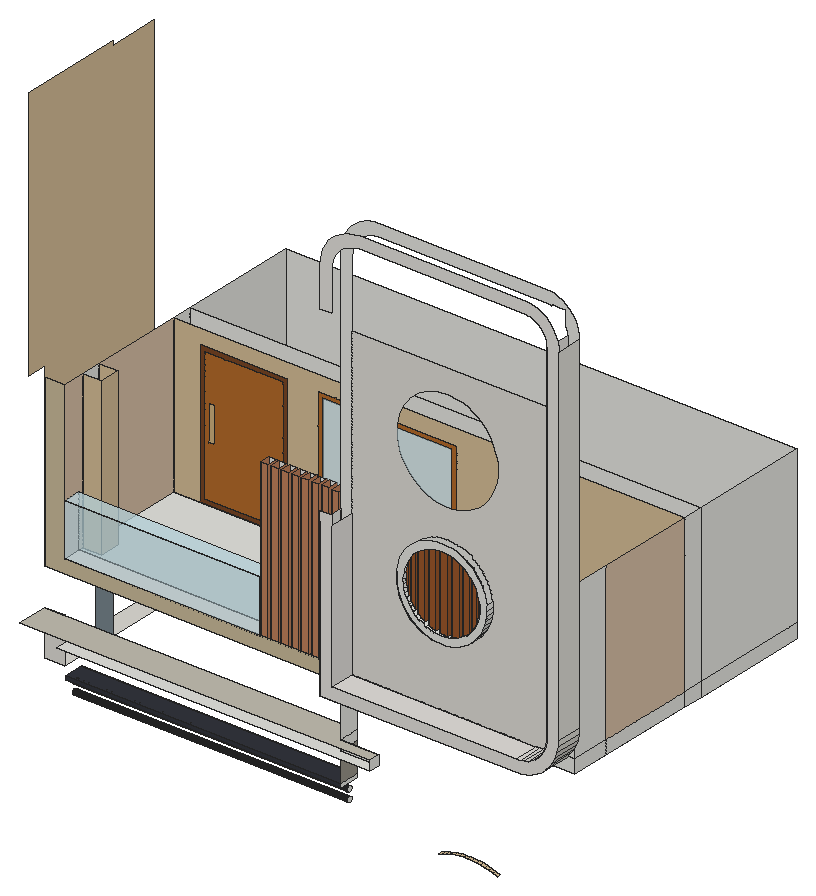
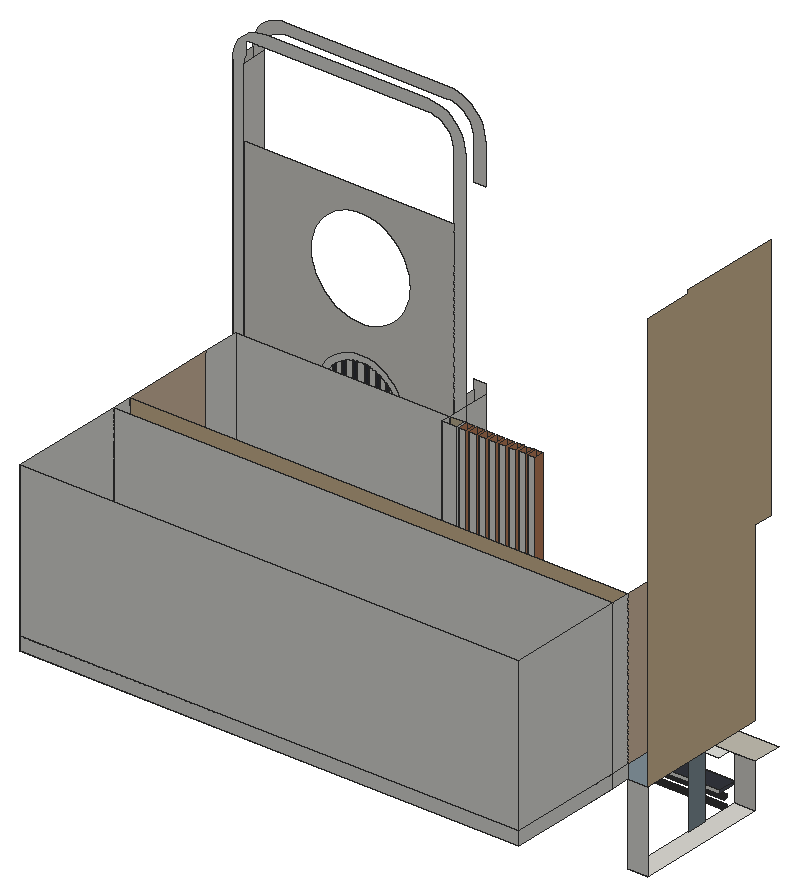
# SketchUp Ruby script. Lengths in inches.
U = 1.inch
M = Sketchup.active_model
def pt(a) = Geom::Point3d.new(a.map { |v| v * U })
def face(e, loops, mat)
  f = e.add_face(loops[0].map { |a| pt(a) })
  loops[1..].each { |l| e.add_face(l.map { |a| pt(a) }).erase! }
  f.material = f.back_material = mat if mat
  f
end
# faces: each face lists its corners as indices into pts; further lists are holes
def faces(e, pts, list, mat = nil) = list.each { |f| face(e, (f[0].is_a?(Array) ? f : [f]).map { |l| l.map { |i| pts[i] } }, mat) }
# xy, xz, yz: faces in a plane at the given z, y or x. An outline is a flat list of corners, or four numbers for a rectangle; further outlines are holes
def ring(l) = l.size == 4 ? [[l[0], l[1]], [l[2], l[1]], [l[2], l[3]], [l[0], l[3]]] : l.each_slice(2).to_a
def flat(e, list, mat, &to3) = list.each { |f| face(e, (f[0].is_a?(Array) ? f : [f]).map { |l| ring(l).map { |u, v| to3.(u, v) } }, mat) }
def xy(e, z, list, mat = nil) = flat(e, list, mat) { |x, y| [x, y, z] }
def xz(e, y, list, mat = nil) = flat(e, list, mat) { |x, z| [x, y, z] }
def yz(e, x, list, mat = nil) = flat(e, list, mat) { |y, z| [x, y, z] }
def lines(e, pts, list) = list.each { |a, b| e.add_line(pt(pts[a]), pt(pts[b])) }
# prism: a flat outline (further loops are holes) pulled along v
def prism(e, loops, v, mat = nil)
  f = face(e, loops, mat); d = Geom::Vector3d.new(v.map { |x| x * U })
  f.pushpull(f.normal.samedirection?(d) ? d.length : -d.length)
end
def box(e, o, s, mat = nil) = prism(e, [[o, [o[0] + s[0], o[1], o[2]], [o[0] + s[0], o[1] + s[1], o[2]], [o[0], o[1] + s[1], o[2]]]], [0, 0, s[2]], mat)
def at(x, y, z, deg = 0) = Geom::Transformation.translation(pt([x, y, z])) * Geom::Transformation.rotation(ORIGIN, Z_AXIS, deg.degrees)
def axes(o, x, y, z) = Geom::Transformation.new([*x, 0, *y, 0, *z, 0, *pt(o).to_a, 1])
def part(name) = M.definitions.add(name)
# library, detail: a bought-in or finely detailed component or shape, given as its bounding box
def library(name, o, s) = part(name).tap { |d| box(d.entities, o, s) }
def detail(e, o, s) = box(e.add_group.entities, o, s)
def put(e, d, t, mat = nil) = e.add_instance(d, t).tap { |i| i.material = mat if mat }
def group(e, t, mat = nil) = e.add_group.tap { |g| g.transformation = t; g.material = mat if mat }.entities
root = M.entities
M.materials.add("[Formica Beige]").color = [211, 187, 149]
M.materials.add("[Formica Graystone]").color = [193, 189, 175]
M.materials.add("[Formica Graystone]1").color = [149, 146, 135]
M.materials.add("[Formica Laminate Dark]").color = [50, 53, 60]
M.materials.add("[Formica Laminate Light]").color = [213, 189, 164]
M.materials.add("[Formica Speckled Grey]").color = [127, 142, 150]
M.materials.add("[Quartz Light Brown]").color = [199, 184, 152]
M.materials.add("[Terrazzo Tile Accent]").color = [224, 221, 217]
M.materials.add("[Terrazzo Tile Light]").color = [219, 217, 210]
M.materials.add("[Translucent Glass Safety]").color = [204, 235, 244]
M.materials["[Translucent Glass Safety]"].alpha = 0.5
M.materials.add("[Wood Bamboo]").color = [177, 105, 43]
M.materials.add("[Wood Cherry Original]").color = [152, 86, 42]
M.materials.add("[Wood Floor Light]").color = [204, 176, 127]
M.materials.add("[Wood Veneer 01]").color = [120, 70, 37]
M.materials.add("[Wood Veneer 02]").color = [190, 128, 91]
xy(root,93.9375,[[0,40.6875,17.9375,162.27]],"[Terrazzo Tile Light]")
xy(root,96.38,[[131.17,22.75,146.95,40.6875],[155.89,22.75,171.0625,40.6875]])
xy(root,96.38,[[32.82,22.75,131.17,40.6875],[171.0625,22.75,277.85,40.6875]],"[Formica Laminate Dark]")
xy(root,99.34,[[32.82,22.75,277.85,40.6875]],"[Formica Laminate Dark]")
xy(root,125.79,[[32.82,13.1875,32.82,40.6875,277.85,40.6875,277.85,22.75,311.48,22.75,311.48,13.1875]])
xy(root,134.5,[[0,13.1875,311.48,13.1875,311.48,22.75,277.85,22.75,277.85,40.6875,0,40.6875]],"[Formica Graystone]")
xy(root,167.375,[[17.9375,75.25,36.375,93.6875],[17.9375,162.27,472.4375,180.28],[17.9375,180.28,472.4375,287.24]])
xy(root,167.375,[[0,40.6875,0,75.25,36.375,75.25,36.375,93.6875,0,93.6875,0,162.27,472.4375,162.27,472.4375,40.6875],[0,75.25,17.9375,93.6875]],"[Formica Speckled Grey]")
xy(root,179.5625,[[277.85,0,451.85,22.75],[17.9375,40.6875,191.93,56.15],[191.93,40.6875,192.74,40.6875,192.74,49.71,277.85,49.71,277.85,56.15,191.93,56.15],[192.74,40.6875,199.15,49.71],[199.15,40.6875,201.68,49.71],
  [201.68,40.6875,208.09,49.71],[208.09,40.6875,210.74,49.71],[210.74,40.6875,217.15,49.71],[217.15,40.6875,219.8,49.71],[219.8,40.6875,226.21,49.71],
  [226.21,40.6875,228.49,49.71],[228.49,40.6875,234.9,49.71],[234.9,40.6875,237.55,49.71],[237.55,40.6875,243.96,49.71],[243.96,40.6875,246.43,49.71],
  [246.43,40.6875,252.84,49.71],[252.84,40.6875,255.74,49.71],[255.74,40.6875,262.15,49.71],[262.15,40.6875,264.27,49.71],[264.27,40.6875,277.85,49.71],
  [277.85,40.6875,472.4375,162.27],[17.9375,56.15,277.85,56.15,277.85,162.27,17.9375,162.27,17.9375,78.66,34.45,78.66,34.45,61.15,17.9375,61.15],[17.9375,61.15,34.45,78.66],[17.9375,162.27,472.4375,180.28],[17.9375,180.28,472.4375,287.24]])
xy(root,179.6875,[[246.43,40.6875,252.84,49.71]])
xy(root,189.9,[[288.19,0,451.85,22.75]],"[Terrazzo Tile Accent]")
xy(root,226.1875,[[17.9375,40.6875,191.93,56.15]],"[Translucent Glass Safety]")
xz(root,0,[[277.85,179.5625,451.85,179.5625,456.88,179.89,461.82,180.875,466.59,182.5,471.11,184.72,475.3,187.52,479.09,190.85,482.41,194.64,485.21,198.83,487.44,203.35,489.0625,208.12,490.05,213.06,490.375,218.09,490.375,527.88,490.12,531.85,489.34,535.76,488.06,539.53,486.3,543.1,484.09,546.41,481.46,549.4,478.47,552.02,475.16,554.24,471.59,556,467.82,557.28,463.92,558.05,459.94,558.3125,312.85,558.3125,308.28,558.01,303.79,557.12,299.46,555.65,295.35,553.625,291.54,551.08,288.1,548.0625,285.08,544.62,282.54,540.8125,280.51,536.71,279.04,532.37,278.15,527.88,277.85,523.3125,277.85,488.3125,288.19,488.3125,288.19,523.3125,288.4,526.53,289.03,529.69,290.07,532.75,291.49,535.64,293.29,538.32,295.41,540.75,297.84,542.875,300.52,544.67,303.41,546.09,306.47,547.13,309.63,547.76,312.85,547.97,459.94,547.97,462.57,547.8,465.14,547.29,467.63,546.44,469.99,545.28,472.18,543.82,474.15,542.09,475.88,540.11,477.34,537.93,478.51,535.57,479.35,533.08,479.86,530.5,480.04,527.88,480.04,218.09,479.79,214.41,479.08,210.79,477.89,207.3,476.26,204,474.21,200.93,471.78,198.16,469.01,195.73,465.94,193.68,462.64,192.05,459.14,190.86,455.53,190.14,451.85,189.9,288.19,189.9,288.19,327.375,277.85,327.375]],"[Terrazzo Tile Accent]")
xz(root,15.8125,[[[373.3125,247.18,377.52,247.4,381.67,248.0625,385.74,249.15,389.67,250.66,393.42,252.57,396.95,254.87,400.23,257.52,403.2,260.49,405.85,263.76,408.14,267.29,410.06,271.05,411.5625,274.98,412.65,279.04,413.3125,283.2,413.53,287.41,413.3125,291.61,412.65,295.77,411.5625,299.83,410.06,303.76,408.14,307.52,405.85,311.05,403.2,314.32,400.23,317.3,396.95,319.94,393.42,322.24,389.67,324.15,385.74,325.66,381.67,326.75,377.52,327.41,373.3125,327.625,369.11,327.41,364.95,326.75,360.88,325.66,356.95,324.15,353.2,322.24,349.67,319.94,346.4,317.3,343.42,314.32,340.77,311.05,338.48,307.52,336.57,303.76,335.06,299.83,333.97,295.77,333.3125,291.61,333.09,287.41,333.3125,283.2,333.97,279.04,335.06,274.98,336.57,271.05,338.48,267.29,340.77,263.76,343.42,260.49,346.4,257.52,349.67,254.87,353.2,252.57,356.95,250.66,360.88,249.15,364.95,248.0625,369.11,247.4],[373.3125,253.375,369.75,253.5625,366.24,254.12,362.8,255.04,359.47,256.32,356.3,257.93,353.31,259.875,350.54,262.12,348.02,264.63,345.78,267.4,343.84,270.39,342.22,273.5625,340.95,276.89,340.02,280.33,339.47,283.85,339.28,287.41,339.47,290.96,340.02,294.48,340.95,297.92,342.22,301.25,343.84,304.42,345.78,307.41,348.02,310.18,350.54,312.7,353.31,314.9375,356.3,316.875,359.47,318.49,362.8,319.77,366.24,320.69,369.75,321.25,373.3125,321.4375,376.87,321.25,380.39,320.69,383.83,319.77,387.15,318.49,390.33,316.875,393.31,314.9375,396.08,312.7,398.6,310.18,400.84,307.41,402.78,304.42,404.4,301.25,405.68,297.92,406.6,294.48,407.16,290.96,407.34,287.41,407.16,283.85,406.6,280.33,405.68,276.89,404.4,273.5625,402.78,270.39,400.84,267.4,398.6,264.63,396.08,262.12,393.31,259.875,390.33,257.93,387.15,256.32,383.83,255.04,380.39,254.12,376.87,253.5625]]])
xz(root,18.4375,[[373.3125,253.375,376.87,253.5625,376.87,321.25,373.3125,321.4375,369.75,321.25,369.75,253.5625],[366.24,254.12,366.24,320.69,362.8,319.77,359.47,318.49,359.47,256.32,362.8,255.04],[380.39,254.12,383.83,255.04,387.15,256.32,387.15,318.49,383.83,319.77,380.39,320.69],[356.3,257.93,356.3,316.875,353.31,314.9375,350.54,312.7,350.54,262.12,353.31,259.875],[390.33,257.93,393.31,259.875,396.08,262.12,396.08,312.7,393.31,314.9375,390.33,316.875],
  [348.02,264.63,348.02,310.18,345.78,307.41,343.84,304.42,343.84,270.39,345.78,267.4],[398.6,264.63,400.84,267.4,402.78,270.39,402.78,304.42,400.84,307.41,398.6,310.18],[342.22,273.5625,342.22,301.25,340.95,297.92,340.02,294.48,339.47,290.96,339.28,287.41,339.47,283.85,340.02,280.33,340.95,276.89],[404.4,273.5625,405.68,276.89,406.6,280.33,407.16,283.85,407.34,287.41,407.16,290.96,406.6,294.48,405.68,297.92,404.4,301.25]],"[Wood Cherry Original]")
xz(root,22.75,[[277.85,125.79,311.48,134.5],[[277.85,179.5625,277.85,523.3125,278.15,527.88,279.04,532.37,280.51,536.71,282.54,540.8125,285.08,544.62,288.1,548.0625,291.54,551.08,295.35,553.625,299.46,555.65,303.79,557.12,308.28,558.01,312.85,558.3125,459.94,558.3125,463.92,558.05,467.82,557.28,471.59,556,475.16,554.24,478.47,552.02,481.46,549.4,484.09,546.41,486.3,543.1,488.06,539.53,489.34,535.76,490.12,531.85,490.375,527.88,490.375,218.09,490.05,213.06,489.0625,208.12,487.44,203.35,485.21,198.83,482.41,194.64,479.09,190.85,475.3,187.52,471.11,184.72,466.59,182.5,461.82,180.875,456.88,179.89,451.85,179.5625],[288.19,189.9,451.85,189.9,455.53,190.14,459.14,190.86,462.64,192.05,465.94,193.68,469.01,195.73,471.78,198.16,474.21,200.93,476.26,204,477.89,207.3,479.08,210.79,479.79,214.41,480.04,218.09,480.04,527.88,479.86,530.5,479.35,533.08,478.51,535.57,478.39,535.8,478.41,544.67,478.41,547.41,476.44,547.8,473.82,547.97,466.08,547.97,466.08,546.97,465.14,547.29,464.53,547.41,464.53,547.97,312.85,547.97,309.63,547.76,306.47,547.13,303.41,546.09,300.52,544.67,297.84,542.875,295.41,540.75,293.29,538.32,291.49,535.64,290.07,532.75,289.03,529.69,288.4,526.53,288.19,523.3125]],[[373.3125,247.18,369.11,247.4,364.95,248.0625,360.88,249.15,356.95,250.66,353.2,252.57,349.67,254.87,346.4,257.52,343.42,260.49,340.77,263.76,338.48,267.29,336.57,271.05,335.06,274.98,333.97,279.04,333.3125,283.2,333.09,287.41,333.3125,291.61,333.97,295.77,335.06,299.83,336.57,303.76,338.48,307.52,340.77,311.05,343.42,314.32,346.4,317.3,349.67,319.94,353.2,322.24,356.95,324.15,360.88,325.66,364.95,326.75,369.11,327.41,373.3125,327.625,377.52,327.41,381.67,326.75,385.74,325.66,389.67,324.15,393.42,322.24,396.95,319.94,400.23,317.3,403.2,314.32,405.85,311.05,408.14,307.52,410.06,303.76,411.5625,299.83,412.65,295.77,413.3125,291.61,413.53,287.41,413.3125,283.2,412.65,279.04,411.5625,274.98,410.06,271.05,408.14,267.29,405.85,263.76,403.2,260.49,400.23,257.52,396.95,254.87,393.42,252.57,389.67,250.66,385.74,249.15,381.67,248.0625,377.52,247.4],[373.3125,253.375,376.87,253.5625,380.39,254.12,383.83,255.04,387.15,256.32,390.33,257.93,393.31,259.875,396.08,262.12,398.6,264.63,400.84,267.4,402.78,270.39,404.4,273.5625,405.68,276.89,406.6,280.33,407.16,283.85,407.34,287.41,407.16,290.96,406.6,294.48,405.68,297.92,404.4,301.25,402.78,304.42,400.84,307.41,398.6,310.18,396.08,312.7,393.31,314.9375,390.33,316.875,387.15,318.49,383.83,319.77,380.39,320.69,376.87,321.25,373.3125,321.4375,369.75,321.25,366.24,320.69,362.8,319.77,359.47,318.49,356.3,316.875,353.31,314.9375,350.54,312.7,348.02,310.18,345.78,307.41,343.84,304.42,342.22,301.25,340.95,297.92,340.02,294.48,339.47,290.96,339.28,287.41,339.47,283.85,340.02,280.33,340.95,276.89,342.22,273.5625,343.84,270.39,345.78,267.4,348.02,264.63,350.54,262.12,353.31,259.875,356.3,257.93,359.47,256.32,362.8,255.04,366.24,254.12,369.75,253.5625]],[373.3125,253.375,369.75,253.5625,369.75,321.25,373.3125,321.4375,376.87,321.25,376.87,253.5625],[366.24,254.12,362.8,255.04,359.47,256.32,359.47,318.49,362.8,319.77,366.24,320.69],
  [380.39,254.12,380.39,320.69,383.83,319.77,387.15,318.49,387.15,256.32,383.83,255.04],[356.3,257.93,353.31,259.875,350.54,262.12,350.54,312.7,353.31,314.9375,356.3,316.875],[390.33,257.93,390.33,316.875,393.31,314.9375,396.08,312.7,396.08,262.12,393.31,259.875],[348.02,264.63,345.78,267.4,343.84,270.39,343.84,304.42,345.78,307.41,348.02,310.18],[398.6,264.63,398.6,310.18,400.84,307.41,402.78,304.42,402.78,270.39,400.84,267.4],
  [342.22,273.5625,340.95,276.89,340.02,280.33,339.47,283.85,339.28,287.41,339.47,290.96,340.02,294.48,340.95,297.92,342.22,301.25],[404.4,273.5625,404.4,301.25,405.68,297.92,406.6,294.48,407.16,290.96,407.34,287.41,407.16,283.85,406.6,280.33,405.68,276.89]])
xz(root,22.75,[[32.82,96.38,277.85,99.34],[369.75,253.5625,369.75,321.25,366.24,320.69,366.24,254.12],[376.87,253.5625,380.39,254.12,380.39,320.69,376.87,321.25],[359.47,256.32,359.47,318.49,356.3,316.875,356.3,257.93],[387.15,256.32,390.33,257.93,390.33,316.875,387.15,318.49],
  [350.54,262.12,350.54,312.7,348.02,310.18,348.02,264.63],[396.08,262.12,398.6,264.63,398.6,310.18,396.08,312.7],[343.84,270.39,343.84,304.42,342.22,301.25,342.22,273.5625],[402.78,270.39,404.4,273.5625,404.4,301.25,402.78,304.42]],"[Formica Laminate Dark]")
xz(root,22.75,[[[288.19,189.9,451.85,189.9,455.53,190.14,459.14,190.86,462.64,192.05,465.94,193.68,469.01,195.73,471.78,198.16,474.21,200.93,476.26,204,477.89,207.3,479.08,210.79,479.79,214.41,480.04,218.09,480.04,464.44,288.19,464.44],[373.3125,352.86,368.57,353.11,363.88,353.85,359.29,355.08,354.86,356.78,350.625,358.9375,346.64,361.53,342.95,364.51,339.59,367.87,336.6,371.5625,334.02,375.55,331.86,379.78,330.16,384.21,328.93,388.8,328.1875,393.49,327.9375,398.23,328.1875,402.98,328.93,407.67,330.16,412.26,331.86,416.69,334.02,420.92,336.6,424.91,339.59,428.6,342.95,431.95,346.64,434.94,350.625,437.53,354.86,439.6875,359.29,441.39,363.88,442.62,368.57,443.36,373.3125,443.61,378.06,443.36,382.75,442.62,387.33,441.39,391.77,439.6875,396,437.53,399.98,434.94,403.67,431.95,407.03,428.6,410.02,424.91,412.61,420.92,414.76,416.69,416.47,412.26,417.7,407.67,418.4375,402.98,418.6875,398.23,418.4375,393.49,417.7,388.8,416.47,384.21,414.76,379.78,412.61,375.55,410.02,371.5625,407.03,367.87,403.67,364.51,399.98,361.53,396,358.9375,391.77,356.78,387.33,355.08,382.75,353.85,378.06,353.11],[373.3125,247.18,369.11,247.4,364.95,248.0625,360.88,249.15,356.95,250.66,353.2,252.57,349.67,254.87,346.4,257.52,343.42,260.49,340.77,263.76,338.48,267.29,336.57,271.05,335.06,274.98,333.97,279.04,333.3125,283.2,333.09,287.41,333.3125,291.61,333.97,295.77,335.06,299.83,336.57,303.76,338.48,307.52,340.77,311.05,343.42,314.32,346.4,317.3,349.67,319.94,353.2,322.24,356.95,324.15,360.88,325.66,364.95,326.75,369.11,327.41,373.3125,327.625,377.52,327.41,381.67,326.75,385.74,325.66,389.67,324.15,393.42,322.24,396.95,319.94,400.23,317.3,403.2,314.32,405.85,311.05,408.14,307.52,410.06,303.76,411.5625,299.83,412.65,295.77,413.3125,291.61,413.53,287.41,413.3125,283.2,412.65,279.04,411.5625,274.98,410.06,271.05,408.14,267.29,405.85,263.76,403.2,260.49,400.23,257.52,396.95,254.87,393.42,252.57,389.67,250.66,385.74,249.15,381.67,248.0625,377.52,247.4]]],"[Terrazzo Tile Light]")
xz(root,40.6875,[[32.82,96.38,277.85,99.34],[277.85,167.375,472.4375,179.5625],[246.43,179.5625,252.84,179.6875],[277.85,179.5625,472.4375,318.5]])
xz(root,40.6875,[[0,167.375,277.85,167.375,277.85,179.5625,17.9375,179.5625,17.9375,318.5,0,318.5],[264.27,179.5625,277.85,318.5]],"[Quartz Light Brown]")
xz(root,40.6875,[[0,93.9375,17.9375,134.5]],"[Terrazzo Tile Light]")
xz(root,40.6875,[[17.9375,179.5625,191.93,226.1875]],"[Translucent Glass Safety]")
xz(root,40.6875,[[192.74,179.5625,199.15,318.5],[201.68,179.5625,208.09,318.5],[210.74,179.5625,217.15,318.5],[219.8,179.5625,226.21,318.5],[228.49,179.5625,234.9,318.5],
  [237.55,179.5625,243.96,318.5],[255.74,179.5625,262.15,318.5],[246.43,179.6875,252.84,318.5]],"[Wood Veneer 02]")
xz(root,49.71,[[192.74,179.5625,199.15,318.5],[201.68,179.5625,208.09,318.5],[210.74,179.5625,217.15,318.5],[219.8,179.5625,226.21,318.5],[228.49,179.5625,234.9,318.5],
  [237.55,179.5625,243.96,318.5],[246.43,179.5625,252.84,179.6875],[255.74,179.5625,262.15,318.5],[264.27,179.5625,277.85,318.5],[246.43,179.6875,252.84,318.5]])
xz(root,56.15,[[17.9375,179.5625,191.93,226.1875]],"[Translucent Glass Safety]")
xz(root,61.15,[[17.9375,179.5625,34.45,318.5]],"[Formica Beige]")
xz(root,78.66,[[17.9375,179.5625,34.45,318.5]],"[Formica Beige]")
xz(root,162.27,[[0,93.9375,17.9375,167.375],[17.9375,167.375,472.4375,179.5625]])
xz(root,162.27,[[[17.9375,179.5625,41.23,179.5625,41.23,305.57,119.1,305.57,119.1,179.5625,472.4375,179.5625,472.4375,318.5,17.9375,318.5],[145.71,193.3,270.09,305.11]]],"[Formica Beige]")
xz(root,162.27,[[150.12,197.71,201.875,300.71],[208.14,197.71,265.68,300.71]],"[Translucent Glass Safety]")
xz(root,162.27,[[[45.63,183.97,114.7,301.16],[49.25,229.85,54,261.48]],[[145.71,193.3,270.09,305.11],[150.12,197.71,265.68,300.71]],[201.875,197.71,208.14,300.71]],"[Wood Bamboo]")
xz(root,162.27,[[49.25,229.85,54,261.48]],"[Wood Floor Light]")
xz(root,162.27,[[[41.23,179.5625,119.1,305.57],[45.63,183.97,114.7,301.16]]],"[Wood Veneer 01]")
xz(root,180.28,[[17.9375,167.375,472.4375,179.5625],[17.9375,179.5625,472.4375,318.5]])
xz(root,287.24,[[17.9375,167.375,472.4375,179.5625],[17.9375,179.5625,472.4375,318.5]])
yz(root,0,[[40.6875,167.375,40.6875,327.375,22.75,327.375,22.75,552.73,116.75,552.73,116.75,549.4375,162.27,549.4375,162.27,167.375]],"[Formica Beige]")
yz(root,17.9375,[[162.27,167.375,180.28,179.5625],[180.28,167.375,287.24,179.5625],[40.6875,179.5625,56.15,226.1875],[61.15,179.5625,78.66,318.5],[162.27,179.5625,180.28,318.5],
  [180.28,179.5625,287.24,318.5]])
yz(root,17.9375,[[56.15,179.5625,61.15,179.5625,61.15,318.5,40.6875,318.5,40.6875,226.1875,56.15,226.1875],[78.66,179.5625,162.27,318.5]],"[Formica Laminate Light]")
yz(root,17.9375,[[75.25,93.9375,93.6875,167.375]],"[Formica Speckled Grey]")
yz(root,34.45,[[61.15,179.5625,78.66,318.5]],"[Formica Beige]")
yz(root,191.93,[[40.6875,179.5625,56.15,226.1875]])
yz(root,192.74,[[40.6875,179.5625,49.71,318.5]],"[Wood Veneer 02]")
yz(root,199.15,[[40.6875,179.5625,49.71,318.5]],"[Wood Veneer 02]")
yz(root,201.68,[[40.6875,179.5625,49.71,318.5]],"[Wood Veneer 02]")
yz(root,208.09,[[40.6875,179.5625,49.71,318.5]],"[Wood Veneer 02]")
yz(root,210.74,[[40.6875,179.5625,49.71,318.5]],"[Wood Veneer 02]")
yz(root,217.15,[[40.6875,179.5625,49.71,318.5]],"[Wood Veneer 02]")
yz(root,219.8,[[40.6875,179.5625,49.71,318.5]],"[Wood Veneer 02]")
yz(root,226.21,[[40.6875,179.5625,49.71,318.5]],"[Wood Veneer 02]")
yz(root,228.49,[[40.6875,179.5625,49.71,318.5]],"[Wood Veneer 02]")
yz(root,234.9,[[40.6875,179.5625,49.71,318.5]],"[Wood Veneer 02]")
yz(root,237.55,[[40.6875,179.5625,49.71,318.5]],"[Wood Veneer 02]")
yz(root,243.96,[[40.6875,179.5625,49.71,318.5]],"[Wood Veneer 02]")
yz(root,246.43,[[40.6875,179.5625,49.71,179.6875]])
yz(root,246.43,[[40.6875,179.6875,49.71,318.5]],"[Wood Veneer 02]")
yz(root,252.84,[[40.6875,179.5625,49.71,179.6875]])
yz(root,252.84,[[40.6875,179.6875,49.71,318.5]],"[Wood Veneer 02]")
yz(root,255.74,[[40.6875,179.5625,49.71,318.5]],"[Wood Veneer 02]")
yz(root,262.15,[[40.6875,179.5625,49.71,318.5]],"[Wood Veneer 02]")
yz(root,264.27,[[40.6875,179.5625,49.71,318.5]])
yz(root,277.85,[[33.12,80.16,33.67,80.24,34.18,80.45,34.62,80.79,34.96,81.23,35.17,81.74,35.24,82.29,35.17,82.84,34.96,83.35,34.62,83.79,34.18,84.13,33.67,84.34,33.12,84.41,32.57,84.34,32.05,84.13,31.61,83.79,31.28,83.35,31.06,82.84,30.99,82.29,31.06,81.74,31.28,81.23,31.61,80.79,32.05,80.45,32.57,80.24],[33.12,88.66,33.67,88.74,34.18,88.95,34.62,89.29,34.96,89.73,35.17,90.24,35.24,90.79,35.17,91.34,34.96,91.85,34.62,92.29,34.18,92.63,33.67,92.84,33.12,92.91,32.57,92.84,32.05,92.63,31.61,92.29,31.28,91.85,31.06,91.34,30.99,90.79,31.06,90.24,31.28,89.73,31.61,89.29,32.05,88.95,32.57,88.74],[22.75,96.38,40.6875,99.34],[22.75,125.79,40.6875,134.5],[22.75,134.5,40.6875,318.5],
  [0,179.5625,22.75,318.5],[40.6875,179.5625,49.71,318.5]])
yz(root,277.85,[[22.75,99.34,40.6875,125.79]],"[Formica Graystone]1")
yz(root,288.19,[[0,189.9,22.75,318.5]],"[Terrazzo Tile Accent]")
yz(root,311.48,[[13.1875,125.79,22.75,134.5]])
yz(root,342.22,[[18.4375,273.5625,22.75,301.25]],"[Wood Cherry Original]")
yz(root,343.84,[[18.4375,270.39,22.75,304.42]],"[Wood Cherry Original]")
yz(root,348.02,[[18.4375,264.63,22.75,310.18]],"[Wood Cherry Original]")
yz(root,350.54,[[18.4375,262.12,22.75,312.7]],"[Wood Cherry Original]")
yz(root,356.3,[[18.4375,257.93,22.75,316.875]],"[Wood Cherry Original]")
yz(root,359.47,[[18.4375,256.32,22.75,318.49]],"[Wood Cherry Original]")
yz(root,366.24,[[18.4375,254.12,22.75,320.69]],"[Wood Cherry Original]")
yz(root,369.75,[[18.4375,253.5625,22.75,321.25]],"[Wood Cherry Original]")
yz(root,376.87,[[18.4375,253.5625,22.75,321.25]],"[Wood Cherry Original]")
yz(root,380.39,[[18.4375,254.12,22.75,320.69]],"[Wood Cherry Original]")
yz(root,387.15,[[18.4375,256.32,22.75,318.49]],"[Wood Cherry Original]")
yz(root,390.33,[[18.4375,257.93,22.75,316.875]],"[Wood Cherry Original]")
yz(root,396.08,[[18.4375,262.12,22.75,312.7]],"[Wood Cherry Original]")
yz(root,398.6,[[18.4375,264.63,22.75,310.18]],"[Wood Cherry Original]")
yz(root,402.78,[[18.4375,270.39,22.75,304.42]],"[Wood Cherry Original]")
yz(root,404.4,[[18.4375,273.5625,22.75,301.25]],"[Wood Cherry Original]")
yz(root,472.4375,[[40.6875,167.375,75.25,179.5625],[75.25,167.375,162.27,179.5625],[162.27,167.375,180.28,179.5625],[180.28,167.375,287.24,179.5625],[40.6875,179.5625,75.25,318.5],
  [162.27,179.5625,180.28,318.5],[180.28,179.5625,287.24,318.5]])
yz(root,472.4375,[[75.25,179.5625,162.27,318.5]],"[Formica Laminate Light]")
yz(root,480.04,[[0,218.09,22.75,527.88]],"[Terrazzo Tile Accent]")
yz(root,490.375,[[0,218.09,22.75,527.88]],"[Terrazzo Tile Light]")
p = [[371.52,22.75,78.01],[367.94,22.75,76.74],[367.94,19.625,76.74],[371.52,19.625,78.01],[419.95,22.75,76.74],[416.37,22.75,78.01],
  [416.37,19.625,78.01],[419.95,19.625,76.74],[375.17,22.75,79.09],[375.17,19.625,79.09],[412.73,22.75,79.09],[412.73,19.625,79.09],
  [378.86,22.75,79.98],[378.86,19.625,79.98],[409.03,22.75,79.98],[409.03,19.625,79.98],[382.59,22.75,80.67],[382.59,19.625,80.67],
  [405.3,22.75,80.67],[405.3,19.625,80.67],[277.85,32.57,80.24],[277.85,32.05,80.45],[32.82,32.05,80.45],[32.82,32.57,80.24],
  [277.85,33.12,80.16],[32.82,33.12,80.16],[277.85,33.67,80.24],[32.82,33.67,80.24],[277.85,34.18,80.45],[32.82,34.18,80.45],
  [277.85,31.61,80.79],[32.82,31.61,80.79],[277.85,34.62,80.79],[32.82,34.62,80.79],[386.36,22.75,81.16],[386.36,19.625,81.16],
  [401.53,22.75,81.16],[401.53,19.625,81.16],[277.85,31.28,81.23],[32.82,31.28,81.23],[277.85,34.96,81.23],[32.82,34.96,81.23],
  [390.15,22.75,81.46],[390.15,19.625,81.46],[397.74,22.75,81.46],[397.74,19.625,81.46],[277.85,31.06,81.74],[32.82,31.06,81.74],
  [277.85,35.17,81.74],[32.82,35.17,81.74],[393.95,22.75,81.5625],[393.95,19.625,81.5625],[277.85,30.99,82.29],[32.82,30.99,82.29],
  [277.85,35.24,82.29],[32.82,35.24,82.29],[277.85,31.06,82.84],[32.82,31.06,82.84],[277.85,35.17,82.84],[32.82,35.17,82.84],
  [277.85,31.28,83.35],[32.82,31.28,83.35],[277.85,34.96,83.35],[32.82,34.96,83.35],[277.85,31.61,83.79],[32.82,31.61,83.79],
  [277.85,34.62,83.79],[32.82,34.62,83.79],[277.85,32.05,84.13],[32.82,32.05,84.13],[277.85,34.18,84.13],[32.82,34.18,84.13],
  [277.85,32.57,84.34],[32.82,32.57,84.34],[277.85,33.67,84.34],[32.82,33.67,84.34],[277.85,33.12,84.41],[32.82,33.12,84.41],
  [277.85,32.57,88.74],[277.85,32.05,88.95],[32.82,32.05,88.95],[32.82,32.57,88.74],[277.85,33.12,88.66],[32.82,33.12,88.66],
  [277.85,33.67,88.74],[32.82,33.67,88.74],[277.85,34.18,88.95],[32.82,34.18,88.95],[277.85,31.61,89.29],[32.82,31.61,89.29],
  [277.85,34.62,89.29],[32.82,34.62,89.29],[277.85,31.28,89.73],[32.82,31.28,89.73],[277.85,34.96,89.73],[32.82,34.96,89.73],
  [277.85,31.06,90.24],[32.82,31.06,90.24],[277.85,35.17,90.24],[32.82,35.17,90.24],[277.85,30.99,90.79],[32.82,30.99,90.79],
  [277.85,35.24,90.79],[32.82,35.24,90.79],[277.85,31.06,91.34],[32.82,31.06,91.34],[277.85,35.17,91.34],[32.82,35.17,91.34],
  [277.85,31.28,91.85],[32.82,31.28,91.85],[277.85,34.96,91.85],[32.82,34.96,91.85],[277.85,31.61,92.29],[32.82,31.61,92.29],
  [277.85,34.62,92.29],[32.82,34.62,92.29],[277.85,32.05,92.63],[32.82,32.05,92.63],[277.85,34.18,92.63],[32.82,34.18,92.63],
  [277.85,32.57,92.84],[32.82,32.57,92.84],[277.85,33.67,92.84],[32.82,33.67,92.84],[277.85,33.12,92.91],[32.82,33.12,92.91],
  [451.85,22.75,179.5625],[456.88,22.75,179.89],[456.88,0,179.89],[451.85,0,179.5625],[461.82,22.75,180.875],[461.82,0,180.875],
  [466.59,22.75,182.5],[466.59,0,182.5],[471.11,22.75,184.72],[471.11,0,184.72],[475.3,22.75,187.52],[475.3,0,187.52],
  [479.09,22.75,190.85],[479.09,0,190.85],[455.53,22.75,190.14],[451.85,22.75,189.9],[451.85,0,189.9],[455.53,0,190.14],
  [459.14,22.75,190.86],[459.14,0,190.86],[482.41,22.75,194.64],[482.41,0,194.64],[462.64,22.75,192.05],[462.64,0,192.05],
  [465.94,22.75,193.68],[465.94,0,193.68],[469.01,22.75,195.73],[469.01,0,195.73],[485.21,22.75,198.83],[485.21,0,198.83],
  [471.78,22.75,198.16],[471.78,0,198.16],[474.21,22.75,200.93],[474.21,0,200.93],[487.44,22.75,203.35],[487.44,0,203.35],
  [476.26,22.75,204],[476.26,0,204],[489.0625,22.75,208.12],[489.0625,0,208.12],[477.89,22.75,207.3],[477.89,0,207.3],
  [479.08,22.75,210.79],[479.08,0,210.79],[490.05,22.75,213.06],[490.05,0,213.06],[479.79,22.75,214.41],[479.79,0,214.41],
  [490.375,22.75,218.09],[490.375,0,218.09],[480.04,22.75,218.09],[480.04,0,218.09],[369.11,22.75,247.4],[373.3125,22.75,247.18],
  [373.3125,15.8125,247.18],[369.11,15.8125,247.4],[377.52,22.75,247.4],[377.52,15.8125,247.4],[364.95,22.75,248.0625],[364.95,15.8125,248.0625],
  [381.67,22.75,248.0625],[381.67,15.8125,248.0625],[360.88,22.75,249.15],[360.88,15.8125,249.15],[385.74,22.75,249.15],[385.74,15.8125,249.15],
  [356.95,22.75,250.66],[356.95,15.8125,250.66],[389.67,22.75,250.66],[389.67,15.8125,250.66],[353.2,22.75,252.57],[353.2,15.8125,252.57],
  [393.42,22.75,252.57],[393.42,15.8125,252.57],[349.67,22.75,254.87],[349.67,15.8125,254.87],[396.95,22.75,254.87],[396.95,15.8125,254.87],
  [373.3125,15.8125,253.375],[373.3125,18.4375,253.375],[369.75,18.4375,253.5625],[369.75,15.8125,253.5625],[376.87,15.8125,253.5625],[376.87,18.4375,253.5625],
  [373.3125,22.75,253.375],[369.75,22.75,253.5625],[376.87,22.75,253.5625],[366.24,22.75,254.12],[366.24,18.4375,254.12],[366.24,15.8125,254.12],
  [380.39,22.75,254.12],[380.39,15.8125,254.12],[380.39,18.4375,254.12],[362.8,18.4375,255.04],[362.8,15.8125,255.04],[383.83,15.8125,255.04],
  [383.83,18.4375,255.04],[362.8,22.75,255.04],[383.83,22.75,255.04],[346.4,22.75,257.52],[346.4,15.8125,257.52],[400.23,22.75,257.52],
  [400.23,15.8125,257.52],[359.47,18.4375,256.32],[359.47,15.8125,256.32],[387.15,15.8125,256.32],[387.15,18.4375,256.32],[359.47,22.75,256.32],
  [387.15,22.75,256.32],[356.3,22.75,257.93],[356.3,18.4375,257.93],[356.3,15.8125,257.93],[390.33,22.75,257.93],[390.33,15.8125,257.93],
  [390.33,18.4375,257.93],[343.42,22.75,260.49],[343.42,15.8125,260.49],[403.2,22.75,260.49],[403.2,15.8125,260.49],[353.31,18.4375,259.875],
  [353.31,15.8125,259.875],[393.31,15.8125,259.875],[393.31,18.4375,259.875],[353.31,22.75,259.875],[393.31,22.75,259.875],[350.54,18.4375,262.12],
  [350.54,15.8125,262.12],[396.08,15.8125,262.12],[396.08,18.4375,262.12],[350.54,22.75,262.12],[396.08,22.75,262.12],[340.77,22.75,263.76],
  [340.77,15.8125,263.76],[405.85,22.75,263.76],[405.85,15.8125,263.76],[348.02,22.75,264.63],[348.02,18.4375,264.63],[348.02,15.8125,264.63],
  [398.6,22.75,264.63],[398.6,15.8125,264.63],[398.6,18.4375,264.63],[338.48,22.75,267.29],[338.48,15.8125,267.29],[408.14,22.75,267.29],
  [408.14,15.8125,267.29],[345.78,18.4375,267.4],[345.78,15.8125,267.4],[400.84,15.8125,267.4],[400.84,18.4375,267.4],[345.78,22.75,267.4],
  [400.84,22.75,267.4],[336.57,22.75,271.05],[336.57,15.8125,271.05],[410.06,22.75,271.05],[410.06,15.8125,271.05],[343.84,18.4375,270.39],
  [343.84,15.8125,270.39],[402.78,15.8125,270.39],[402.78,18.4375,270.39],[343.84,22.75,270.39],[402.78,22.75,270.39],[342.22,22.75,273.5625],
  [342.22,18.4375,273.5625],[342.22,15.8125,273.5625],[404.4,22.75,273.5625],[404.4,15.8125,273.5625],[404.4,18.4375,273.5625],[335.06,22.75,274.98],
  [335.06,15.8125,274.98],[411.5625,22.75,274.98],[411.5625,15.8125,274.98],[340.95,18.4375,276.89],[340.95,15.8125,276.89],[405.68,15.8125,276.89],
  [405.68,18.4375,276.89],[340.95,22.75,276.89],[405.68,22.75,276.89],[333.97,22.75,279.04],[333.97,15.8125,279.04],[412.65,22.75,279.04],
  [412.65,15.8125,279.04],[340.02,18.4375,280.33],[340.02,15.8125,280.33],[406.6,15.8125,280.33],[406.6,18.4375,280.33],[340.02,22.75,280.33],
  [406.6,22.75,280.33],[333.3125,22.75,283.2],[333.3125,15.8125,283.2],[413.3125,22.75,283.2],[413.3125,15.8125,283.2],[339.47,18.4375,283.85],
  [339.47,15.8125,283.85],[407.16,15.8125,283.85],[407.16,18.4375,283.85],[339.47,22.75,283.85],[407.16,22.75,283.85],[333.09,22.75,287.41],
  [333.09,15.8125,287.41],[413.53,22.75,287.41],[413.53,15.8125,287.41],[339.28,18.4375,287.41],[339.28,15.8125,287.41],[407.34,15.8125,287.41],
  [407.34,18.4375,287.41],[339.28,22.75,287.41],[407.34,22.75,287.41],[333.3125,22.75,291.61],[333.3125,15.8125,291.61],[339.47,18.4375,290.96],
  [339.47,15.8125,290.96],[407.16,15.8125,290.96],[407.16,18.4375,290.96],[413.3125,22.75,291.61],[413.3125,15.8125,291.61],[339.47,22.75,290.96],
  [407.16,22.75,290.96]]
faces(root,p,[[0,1,2,3],[4,5,6,7],[8,0,3,9],[5,10,11,6],[12,8,9,13],[10,14,15,11],[16,12,13,17],[14,18,19,15],
  [34,16,17,35],[18,36,37,19],[42,34,35,43],[36,44,45,37],[50,42,43,51],[44,50,51,45]],"[Formica Beige]")
faces(root,p,[[20,21,22,23],[24,20,23,25],[26,24,25,27],[28,26,27,29],[21,30,31,22],[32,28,29,33],[30,38,39,31],[40,32,33,41],
  [38,46,47,39],[48,40,41,49],[46,52,53,47],[54,48,49,55],[52,56,57,53],[58,54,55,59],[56,60,61,57],[62,58,59,63],
  [60,64,65,61],[66,62,63,67],[64,68,69,65],[70,66,67,71],[68,72,73,69],[74,70,71,75],[72,76,77,73],[76,74,75,77],
  [78,79,80,81],[82,78,81,83],[84,82,83,85],[86,84,85,87],[79,88,89,80],[90,86,87,91],[88,92,93,89],[94,90,91,95],
  [92,96,97,93],[98,94,95,99],[96,100,101,97],[102,98,99,103],[100,104,105,101],[106,102,103,107],[104,108,109,105],[110,106,107,111],
  [108,112,113,109],[114,110,111,115],[112,116,117,113],[118,114,115,119],[116,120,121,117],[122,118,119,123],[120,124,125,121],[124,122,123,125]],"[Formica Laminate Dark]")
faces(root,p,[[126,127,128,129],[127,130,131,128],[130,132,133,131],[132,134,135,133],[134,136,137,135],[136,138,139,137],[138,146,147,139],[146,154,155,147],
  [154,160,161,155],[160,164,165,161],[164,170,171,165],[170,174,175,171]],"[Terrazzo Tile Light]")
faces(root,p,[[140,141,142,143],[144,140,143,145],[148,144,145,149],[150,148,149,151],[152,150,151,153],[156,152,153,157],[158,156,157,159],[162,158,159,163],
  [166,162,163,167],[168,166,167,169],[172,168,169,173],[176,172,173,177]],"[Terrazzo Tile Accent]")
faces(root,p,[[178,179,180,181],[179,182,183,180],[184,178,181,185],[182,186,187,183],[188,184,185,189],[186,190,191,187],[192,188,189,193],[190,194,195,191],
  [196,192,193,197],[194,198,199,195],[200,196,197,201],[198,202,203,199],[204,205,206,207],[208,209,205,204],[210,211,206,205],[212,210,205,209],
  [211,213,214,215,207,206],[216,212,209,208,217,218],[215,214,219,220],[221,222,218,217],[213,223,219,214],[224,216,218,222],[225,200,201,226],[202,227,228,203],
  [220,219,229,230],[231,232,222,221],[223,233,229,219],[234,224,222,232],[233,235,236,237,230,229],[238,234,232,231,239,240],[241,225,226,242],[227,243,244,228],
  [237,236,245,246],[247,248,240,239],[235,249,245,236],[250,238,240,248],[246,245,251,252],[253,254,248,247],[249,255,251,245],[256,250,248,254],
  [257,241,242,258],[243,259,260,244],[255,261,262,263,252,251],[264,256,254,253,265,266],[267,257,258,268],[259,269,270,260],[263,262,271,272],[273,274,266,265],
  [261,275,271,262],[276,264,266,274],[277,267,268,278],[269,279,280,270],[272,271,281,282],[283,284,274,273],[275,285,281,271],[286,276,274,284],
  [285,287,288,289,282,281],[290,286,284,283,291,292],[293,277,278,294],[279,295,296,280],[289,288,297,298],[299,300,292,291],[287,301,297,288],[302,290,292,300],
  [303,293,294,304],[295,305,306,296],[298,297,307,308],[309,310,300,299],[301,311,307,297],[312,302,300,310],[313,303,304,314],[305,315,316,306],
  [308,307,317,318],[319,320,310,309],[311,321,317,307],[322,312,310,320],[323,313,314,324],[315,325,326,316],[318,317,327,328],[329,330,320,319],
  [321,331,327,317],[332,322,320,330],[333,323,324,334],[328,327,335,336],[337,338,330,329],[325,339,340,326],[331,341,335,327],[342,332,330,338]])
